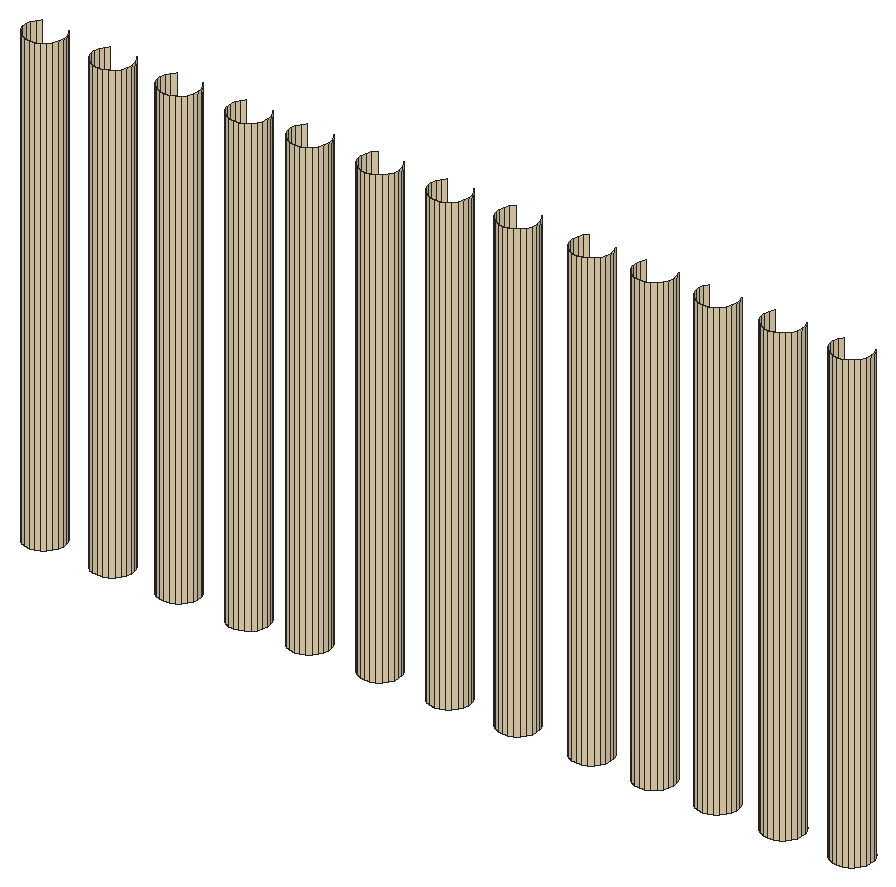
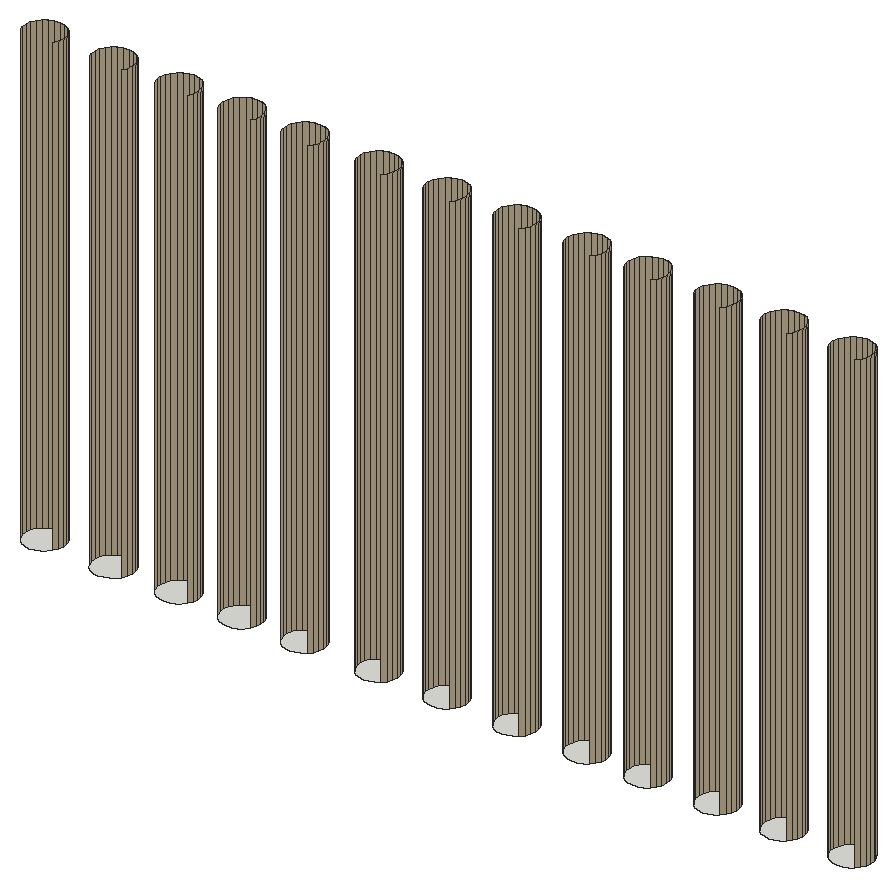
# SketchUp Ruby script. Lengths in inches.
U = 1.inch
M = Sketchup.active_model
def pt(a) = Geom::Point3d.new(a.map { |v| v * U })
def face(e, loops, mat)
  f = e.add_face(loops[0].map { |a| pt(a) })
  loops[1..].each { |l| e.add_face(l.map { |a| pt(a) }).erase! }
  f.material = f.back_material = mat if mat
  f
end
# faces: each face lists its corners as indices into pts; further lists are holes
def faces(e, pts, list, mat = nil) = list.each { |f| face(e, (f[0].is_a?(Array) ? f : [f]).map { |l| l.map { |i| pts[i] } }, mat) }
# xy, xz, yz: faces in a plane at the given z, y or x. An outline is a flat list of corners, or four numbers for a rectangle; further outlines are holes
def ring(l) = l.size == 4 ? [[l[0], l[1]], [l[2], l[1]], [l[2], l[3]], [l[0], l[3]]] : l.each_slice(2).to_a
def flat(e, list, mat, &to3) = list.each { |f| face(e, (f[0].is_a?(Array) ? f : [f]).map { |l| ring(l).map { |u, v| to3.(u, v) } }, mat) }
def xy(e, z, list, mat = nil) = flat(e, list, mat) { |x, y| [x, y, z] }
def xz(e, y, list, mat = nil) = flat(e, list, mat) { |x, z| [x, y, z] }
def yz(e, x, list, mat = nil) = flat(e, list, mat) { |y, z| [x, y, z] }
def lines(e, pts, list) = list.each { |a, b| e.add_line(pt(pts[a]), pt(pts[b])) }
# prism: a flat outline (further loops are holes) pulled along v
def prism(e, loops, v, mat = nil)
  f = face(e, loops, mat); d = Geom::Vector3d.new(v.map { |x| x * U })
  f.pushpull(f.normal.samedirection?(d) ? d.length : -d.length)
end
def box(e, o, s, mat = nil) = prism(e, [[o, [o[0] + s[0], o[1], o[2]], [o[0] + s[0], o[1] + s[1], o[2]], [o[0], o[1] + s[1], o[2]]]], [0, 0, s[2]], mat)
def at(x, y, z, deg = 0) = Geom::Transformation.translation(pt([x, y, z])) * Geom::Transformation.rotation(ORIGIN, Z_AXIS, deg.degrees)
def axes(o, x, y, z) = Geom::Transformation.new([*x, 0, *y, 0, *z, 0, *pt(o).to_a, 1])
def part(name) = M.definitions.add(name)
# library, detail: a bought-in or finely detailed component or shape, given as its bounding box
def library(name, o, s) = part(name).tap { |d| box(d.entities, o, s) }
def detail(e, o, s) = box(e.add_group.entities, o, s)
def put(e, d, t, mat = nil) = e.add_instance(d, t).tap { |i| i.material = mat if mat }
def group(e, t, mat = nil) = e.add_group.tap { |g| g.transformation = t; g.material = mat if mat }.entities
root = M.entities
M.materials.add("[Quartz Light Brown]").color = [242, 223, 185]
xy(root,566.75,[[491.82,18.95,491.37,19.01,490.94,19.18,490.58,19.46,490.3,19.83,490.13,20.25,490.07,20.7,490.13,21.15,490.3,21.58,490.58,21.9375,490.94,22.22,491.37,22.39,491.82,22.45,492.27,22.39,492.69,22.22,493.06,21.9375,493.33,21.58,493.51,21.15,493.57,20.7,493.51,20.25,493.33,19.83,493.06,19.46,492.69,19.18,492.27,19.01],[498.13,18.95,497.68,19.01,497.26,19.18,496.89,19.46,496.62,19.83,496.44,20.25,496.38,20.7,496.44,21.15,496.62,21.58,496.89,21.9375,497.26,22.22,497.68,22.39,498.13,22.45,498.58,22.39,499.01,22.22,499.37,21.9375,499.65,21.58,499.82,21.15,499.88,20.7,499.82,20.25,499.65,19.83,499.37,19.46,499.01,19.18,498.58,19.01],[504.26,18.95,503.8,19.01,503.38,19.18,503.02,19.46,502.74,19.83,502.57,20.25,502.51,20.7,502.57,21.15,502.74,21.58,503.02,21.9375,503.38,22.22,503.8,22.39,504.26,22.45,504.71,22.39,505.13,22.22,505.49,21.9375,505.77,21.58,505.95,21.15,506.01,20.7,505.95,20.25,505.77,19.83,505.49,19.46,505.13,19.18,504.71,19.01],[510.69,18.95,510.24,19.01,509.82,19.18,509.46,19.46,509.18,19.83,509,20.25,508.94,20.7,509,21.15,509.18,21.58,509.46,21.9375,509.82,22.22,510.24,22.39,510.69,22.45,511.15,22.39,511.57,22.22,511.93,21.9375,512.21,21.58,512.38,21.15,512.44,20.7,512.38,20.25,512.21,19.83,511.93,19.46,511.57,19.18,511.15,19.01],[516.32,18.95,515.87,19.01,515.44,19.18,515.08,19.46,514.8,19.83,514.63,20.25,514.57,20.7,514.63,21.15,514.8,21.58,515.08,21.9375,515.44,22.22,515.87,22.39,516.32,22.45,516.77,22.39,517.19,22.22,517.56,21.9375,517.83,21.58,518.01,21.15,518.07,20.7,518.01,20.25,517.83,19.83,517.56,19.46,517.19,19.18,516.77,19.01],
  [522.82,18.95,522.37,19.01,521.94,19.18,521.58,19.46,521.3,19.83,521.13,20.25,521.07,20.7,521.13,21.15,521.3,21.58,521.58,21.9375,521.94,22.22,522.37,22.39,522.82,22.45,523.27,22.39,523.69,22.22,524.06,21.9375,524.33,21.58,524.51,21.15,524.57,20.7,524.51,20.25,524.33,19.83,524.06,19.46,523.69,19.18,523.27,19.01],[529.26,18.95,528.8,19.01,528.38,19.18,528.02,19.46,527.74,19.83,527.57,20.25,527.51,20.7,527.57,21.15,527.74,21.58,528.02,21.9375,528.38,22.22,528.8,22.39,529.26,22.45,529.71,22.39,530.13,22.22,530.49,21.9375,530.77,21.58,530.95,21.15,531.01,20.7,530.95,20.25,530.77,19.83,530.49,19.46,530.13,19.18,529.71,19.01],[535.57,18.95,535.12,19.01,534.69,19.18,534.33,19.46,534.05,19.83,533.88,20.25,533.82,20.7,533.88,21.15,534.05,21.58,534.33,21.9375,534.69,22.22,535.12,22.39,535.57,22.45,536.02,22.39,536.44,22.22,536.81,21.9375,537.08,21.58,537.26,21.15,537.32,20.7,537.26,20.25,537.08,19.83,536.81,19.46,536.44,19.18,536.02,19.01],[542.38,18.95,541.93,19.01,541.51,19.18,541.14,19.46,540.87,19.83,540.69,20.25,540.63,20.7,540.69,21.15,540.87,21.58,541.14,21.9375,541.51,22.22,541.93,22.39,542.38,22.45,542.83,22.39,543.26,22.22,543.62,21.9375,543.9,21.58,544.07,21.15,544.13,20.7,544.07,20.25,543.9,19.83,543.62,19.46,543.26,19.18,542.83,19.01],[548.19,18.95,547.74,19.01,547.32,19.18,546.96,19.46,546.68,19.83,546.5,20.25,546.44,20.7,546.5,21.15,546.68,21.58,546.96,21.9375,547.32,22.22,547.74,22.39,548.19,22.45,548.65,22.39,549.07,22.22,549.43,21.9375,549.71,21.58,549.88,21.15,549.94,20.7,549.88,20.25,549.71,19.83,549.43,19.46,549.07,19.18,548.65,19.01],
  [554.01,18.95,553.55,19.01,553.13,19.18,552.77,19.46,552.49,19.83,552.32,20.25,552.26,20.7,552.32,21.15,552.49,21.58,552.77,21.9375,553.13,22.22,553.55,22.39,554.01,22.45,554.46,22.39,554.88,22.22,555.24,21.9375,555.52,21.58,555.7,21.15,555.76,20.7,555.7,20.25,555.52,19.83,555.24,19.46,554.88,19.18,554.46,19.01],[560.07,18.95,559.62,19.01,559.19,19.18,558.83,19.46,558.55,19.83,558.38,20.25,558.32,20.7,558.38,21.15,558.55,21.58,558.83,21.9375,559.19,22.22,559.62,22.39,560.07,22.45,560.52,22.39,560.94,22.22,561.31,21.9375,561.58,21.58,561.76,21.15,561.82,20.7,561.76,20.25,561.58,19.83,561.31,19.46,560.94,19.18,560.52,19.01],[566.44,18.95,565.99,19.01,565.57,19.18,565.21,19.46,564.93,19.83,564.75,20.25,564.69,20.7,564.75,21.15,564.93,21.58,565.21,21.9375,565.57,22.22,565.99,22.39,566.44,22.45,566.9,22.39,567.32,22.22,567.68,21.9375,567.96,21.58,568.13,21.15,568.19,20.7,568.13,20.25,567.96,19.83,567.68,19.46,567.32,19.18,566.9,19.01]])
p = [[490.94,19.18,566.75],[491.37,19.01,566.75],[491.37,19.01,608.75],[490.94,19.18,608.75],[491.82,18.95,566.75],[491.82,18.95,608.75],
  [492.27,19.01,566.75],[492.27,19.01,608.75],[492.69,19.18,566.75],[492.69,19.18,608.75],[497.26,19.18,566.75],[497.68,19.01,566.75],
  [497.68,19.01,608.75],[497.26,19.18,608.75],[498.13,18.95,566.75],[498.13,18.95,608.75],[498.58,19.01,566.75],[498.58,19.01,608.75],
  [499.01,19.18,566.75],[499.01,19.18,608.75],[503.38,19.18,566.75],[503.8,19.01,566.75],[503.8,19.01,608.75],[503.38,19.18,608.75],
  [504.26,18.95,566.75],[504.26,18.95,608.75],[504.71,19.01,566.75],[504.71,19.01,608.75],[505.13,19.18,566.75],[505.13,19.18,608.75],
  [509.82,19.18,566.75],[510.24,19.01,566.75],[510.24,19.01,608.75],[509.82,19.18,608.75],[510.69,18.95,566.75],[510.69,18.95,608.75],
  [511.15,19.01,566.75],[511.15,19.01,608.75],[511.57,19.18,566.75],[511.57,19.18,608.75],[515.44,19.18,566.75],[515.87,19.01,566.75],
  [515.87,19.01,608.75],[515.44,19.18,608.75],[516.32,18.95,566.75],[516.32,18.95,608.75],[516.77,19.01,566.75],[516.77,19.01,608.75],
  [517.19,19.18,566.75],[517.19,19.18,608.75],[521.94,19.18,566.75],[522.37,19.01,566.75],[522.37,19.01,608.75],[521.94,19.18,608.75],
  [522.82,18.95,566.75],[522.82,18.95,608.75],[523.27,19.01,566.75],[523.27,19.01,608.75],[523.69,19.18,566.75],[523.69,19.18,608.75],
  [528.38,19.18,566.75],[528.8,19.01,566.75],[528.8,19.01,608.75],[528.38,19.18,608.75],[529.26,18.95,566.75],[529.26,18.95,608.75],
  [529.71,19.01,566.75],[529.71,19.01,608.75],[530.13,19.18,566.75],[530.13,19.18,608.75],[534.69,19.18,566.75],[535.12,19.01,566.75],
  [535.12,19.01,608.75],[534.69,19.18,608.75],[535.57,18.95,566.75],[535.57,18.95,608.75],[536.02,19.01,566.75],[536.02,19.01,608.75],
  [536.44,19.18,566.75],[536.44,19.18,608.75],[541.51,19.18,566.75],[541.93,19.01,566.75],[541.93,19.01,608.75],[541.51,19.18,608.75],
  [542.38,18.95,566.75],[542.38,18.95,608.75],[542.83,19.01,566.75],[542.83,19.01,608.75],[543.26,19.18,566.75],[543.26,19.18,608.75],
  [547.32,19.18,566.75],[547.74,19.01,566.75],[547.74,19.01,608.75],[547.32,19.18,608.75],[548.19,18.95,566.75],[548.19,18.95,608.75],
  [548.65,19.01,566.75],[548.65,19.01,608.75],[549.07,19.18,566.75],[549.07,19.18,608.75],[553.13,19.18,566.75],[553.55,19.01,566.75],
  [553.55,19.01,608.75],[553.13,19.18,608.75],[554.01,18.95,566.75],[554.01,18.95,608.75],[554.46,19.01,566.75],[554.46,19.01,608.75],
  [554.88,19.18,566.75],[554.88,19.18,608.75],[559.19,19.18,566.75],[559.62,19.01,566.75],[559.62,19.01,608.75],[559.19,19.18,608.75],
  [560.07,18.95,566.75],[560.07,18.95,608.75],[560.52,19.01,566.75],[560.52,19.01,608.75],[560.94,19.18,566.75],[560.94,19.18,608.75],
  [565.57,19.18,566.75],[565.99,19.01,566.75],[565.99,19.01,608.75],[565.57,19.18,608.75],[566.44,18.95,566.75],[566.44,18.95,608.75],
  [566.9,19.01,566.75],[566.9,19.01,608.75],[567.32,19.18,566.75],[567.32,19.18,608.75],[490.58,19.46,566.75],[490.58,19.46,608.75],
  [493.06,19.46,566.75],[493.06,19.46,608.75],[496.89,19.46,566.75],[496.89,19.46,608.75],[499.37,19.46,566.75],[499.37,19.46,608.75],
  [503.02,19.46,566.75],[503.02,19.46,608.75],[505.49,19.46,566.75],[505.49,19.46,608.75],[509.46,19.46,566.75],[509.46,19.46,608.75],
  [511.93,19.46,566.75],[511.93,19.46,608.75],[515.08,19.46,566.75],[515.08,19.46,608.75],[517.56,19.46,566.75],[517.56,19.46,608.75],
  [521.58,19.46,566.75],[521.58,19.46,608.75],[524.06,19.46,566.75],[524.06,19.46,608.75],[528.02,19.46,566.75],[528.02,19.46,608.75],
  [530.49,19.46,566.75],[530.49,19.46,608.75],[534.33,19.46,566.75],[534.33,19.46,608.75],[536.81,19.46,566.75],[536.81,19.46,608.75],
  [541.14,19.46,566.75],[541.14,19.46,608.75],[543.62,19.46,566.75],[543.62,19.46,608.75],[546.96,19.46,566.75],[546.96,19.46,608.75],
  [549.43,19.46,566.75],[549.43,19.46,608.75],[552.77,19.46,566.75],[552.77,19.46,608.75],[555.24,19.46,566.75],[555.24,19.46,608.75],
  [558.83,19.46,566.75],[558.83,19.46,608.75],[561.31,19.46,566.75],[561.31,19.46,608.75],[565.21,19.46,566.75],[565.21,19.46,608.75],
  [567.68,19.46,566.75],[567.68,19.46,608.75],[490.3,19.83,566.75],[490.3,19.83,608.75],[493.33,19.83,566.75],[493.33,19.83,608.75],
  [496.62,19.83,566.75],[496.62,19.83,608.75],[499.65,19.83,566.75],[499.65,19.83,608.75],[502.74,19.83,566.75],[502.74,19.83,608.75],
  [505.77,19.83,566.75],[505.77,19.83,608.75],[509.18,19.83,566.75],[509.18,19.83,608.75],[512.21,19.83,566.75],[512.21,19.83,608.75],
  [514.8,19.83,566.75],[514.8,19.83,608.75],[517.83,19.83,566.75],[517.83,19.83,608.75],[521.3,19.83,566.75],[521.3,19.83,608.75],
  [524.33,19.83,566.75],[524.33,19.83,608.75],[527.74,19.83,566.75],[527.74,19.83,608.75],[530.77,19.83,566.75],[530.77,19.83,608.75],
  [534.05,19.83,566.75],[534.05,19.83,608.75],[537.08,19.83,566.75],[537.08,19.83,608.75],[540.87,19.83,566.75],[540.87,19.83,608.75],
  [543.9,19.83,566.75],[543.9,19.83,608.75],[546.68,19.83,566.75],[546.68,19.83,608.75],[549.71,19.83,566.75],[549.71,19.83,608.75],
  [552.49,19.83,566.75],[552.49,19.83,608.75],[555.52,19.83,566.75],[555.52,19.83,608.75],[558.55,19.83,566.75],[558.55,19.83,608.75],
  [561.58,19.83,566.75],[561.58,19.83,608.75],[564.93,19.83,566.75],[564.93,19.83,608.75],[567.96,19.83,566.75],[567.96,19.83,608.75],
  [490.13,20.25,566.75],[490.13,20.25,608.75],[493.51,20.25,566.75],[493.51,20.25,608.75],[496.44,20.25,566.75],[496.44,20.25,608.75],
  [499.82,20.25,566.75],[499.82,20.25,608.75],[502.57,20.25,566.75],[502.57,20.25,608.75],[505.95,20.25,566.75],[505.95,20.25,608.75],
  [509,20.25,566.75],[509,20.25,608.75],[512.38,20.25,566.75],[512.38,20.25,608.75],[514.63,20.25,566.75],[514.63,20.25,608.75],
  [518.01,20.25,566.75],[518.01,20.25,608.75],[521.13,20.25,566.75],[521.13,20.25,608.75],[524.51,20.25,566.75],[524.51,20.25,608.75],
  [527.57,20.25,566.75],[527.57,20.25,608.75],[530.95,20.25,566.75],[530.95,20.25,608.75],[533.88,20.25,566.75],[533.88,20.25,608.75],
  [537.26,20.25,566.75],[537.26,20.25,608.75],[540.69,20.25,566.75],[540.69,20.25,608.75],[544.07,20.25,566.75],[544.07,20.25,608.75],
  [546.5,20.25,566.75],[546.5,20.25,608.75],[549.88,20.25,566.75],[549.88,20.25,608.75],[552.32,20.25,566.75],[552.32,20.25,608.75],
  [555.7,20.25,566.75],[555.7,20.25,608.75],[558.38,20.25,566.75],[558.38,20.25,608.75],[561.76,20.25,566.75],[561.76,20.25,608.75],
  [564.75,20.25,566.75],[564.75,20.25,608.75],[568.13,20.25,566.75],[568.13,20.25,608.75],[490.07,20.7,566.75],[490.07,20.7,608.75],
  [493.57,20.7,566.75],[493.57,20.7,608.75],[496.38,20.7,566.75],[496.38,20.7,608.75],[499.88,20.7,566.75],[499.88,20.7,608.75],
  [502.51,20.7,566.75],[502.51,20.7,608.75],[506.01,20.7,566.75],[506.01,20.7,608.75],[508.94,20.7,566.75],[508.94,20.7,608.75],
  [512.44,20.7,566.75],[512.44,20.7,608.75],[514.57,20.7,566.75],[514.57,20.7,608.75],[518.07,20.7,566.75],[518.07,20.7,608.75],
  [521.07,20.7,566.75],[521.07,20.7,608.75],[524.57,20.7,566.75],[524.57,20.7,608.75],[527.51,20.7,566.75],[527.51,20.7,608.75],
  [531.01,20.7,566.75],[531.01,20.7,608.75],[533.82,20.7,566.75],[533.82,20.7,608.75],[537.32,20.7,566.75],[537.32,20.7,608.75],
  [540.63,20.7,566.75],[540.63,20.7,608.75],[544.13,20.7,566.75],[544.13,20.7,608.75],[546.44,20.7,566.75],[546.44,20.7,608.75],
  [549.94,20.7,566.75],[549.94,20.7,608.75],[552.26,20.7,566.75],[552.26,20.7,608.75],[555.76,20.7,566.75],[555.76,20.7,608.75],
  [558.32,20.7,566.75],[558.32,20.7,608.75],[561.82,20.7,566.75],[561.82,20.7,608.75],[564.69,20.7,566.75],[564.69,20.7,608.75],
  [568.19,20.7,566.75],[568.19,20.7,608.75],[490.13,21.15,566.75],[490.13,21.15,608.75],[493.51,21.15,566.75],[493.51,21.15,608.75],
  [496.44,21.15,566.75],[496.44,21.15,608.75],[499.82,21.15,566.75],[499.82,21.15,608.75],[502.57,21.15,566.75],[502.57,21.15,608.75],
  [505.95,21.15,566.75],[505.95,21.15,608.75],[509,21.15,566.75],[509,21.15,608.75],[512.38,21.15,566.75],[512.38,21.15,608.75],
  [514.63,21.15,566.75],[514.63,21.15,608.75],[518.01,21.15,566.75],[518.01,21.15,608.75],[521.13,21.15,566.75],[521.13,21.15,608.75],
  [524.51,21.15,566.75],[524.51,21.15,608.75],[527.57,21.15,566.75],[527.57,21.15,608.75],[530.95,21.15,566.75],[530.95,21.15,608.75],
  [533.88,21.15,566.75],[533.88,21.15,608.75],[537.26,21.15,566.75],[537.26,21.15,608.75],[540.69,21.15,566.75],[540.69,21.15,608.75],
  [544.07,21.15,566.75],[544.07,21.15,608.75],[546.5,21.15,566.75],[546.5,21.15,608.75],[549.88,21.15,566.75],[549.88,21.15,608.75],
  [552.32,21.15,566.75],[552.32,21.15,608.75],[555.7,21.15,566.75],[555.7,21.15,608.75],[558.38,21.15,566.75],[558.38,21.15,608.75],
  [561.76,21.15,566.75],[561.76,21.15,608.75],[564.75,21.15,566.75],[564.75,21.15,608.75],[568.13,21.15,566.75],[568.13,21.15,608.75],
  [490.3,21.58,566.75],[490.3,21.58,608.75],[493.33,21.58,566.75],[493.33,21.58,608.75],[496.62,21.58,566.75],[496.62,21.58,608.75],
  [499.65,21.58,566.75],[499.65,21.58,608.75],[502.74,21.58,566.75],[502.74,21.58,608.75],[505.77,21.58,566.75],[505.77,21.58,608.75],
  [509.18,21.58,566.75],[509.18,21.58,608.75],[512.21,21.58,566.75],[512.21,21.58,608.75],[514.8,21.58,566.75],[514.8,21.58,608.75],
  [517.83,21.58,566.75],[517.83,21.58,608.75],[521.3,21.58,566.75],[521.3,21.58,608.75],[524.33,21.58,566.75],[524.33,21.58,608.75],
  [527.74,21.58,566.75],[527.74,21.58,608.75],[530.77,21.58,566.75],[530.77,21.58,608.75],[534.05,21.58,566.75],[534.05,21.58,608.75],
  [537.08,21.58,566.75],[537.08,21.58,608.75],[540.87,21.58,566.75],[540.87,21.58,608.75],[543.9,21.58,566.75],[543.9,21.58,608.75],
  [546.68,21.58,566.75],[546.68,21.58,608.75],[549.71,21.58,566.75],[549.71,21.58,608.75],[552.49,21.58,566.75],[552.49,21.58,608.75],
  [555.52,21.58,566.75],[555.52,21.58,608.75],[558.55,21.58,566.75],[558.55,21.58,608.75],[561.58,21.58,566.75],[561.58,21.58,608.75],
  [564.93,21.58,566.75],[564.93,21.58,608.75],[567.96,21.58,566.75],[567.96,21.58,608.75],[490.58,21.9375,566.75],[490.58,21.9375,608.75],
  [493.06,21.9375,566.75],[493.06,21.9375,608.75],[496.89,21.9375,566.75],[496.89,21.9375,608.75],[499.37,21.9375,566.75],[499.37,21.9375,608.75],
  [503.02,21.9375,566.75],[503.02,21.9375,608.75],[505.49,21.9375,566.75],[505.49,21.9375,608.75],[509.46,21.9375,566.75],[509.46,21.9375,608.75],
  [511.93,21.9375,566.75],[511.93,21.9375,608.75],[515.08,21.9375,566.75],[515.08,21.9375,608.75],[517.56,21.9375,566.75],[517.56,21.9375,608.75],
  [521.58,21.9375,566.75],[521.58,21.9375,608.75],[524.06,21.9375,566.75],[524.06,21.9375,608.75],[528.02,21.9375,566.75],[528.02,21.9375,608.75],
  [530.49,21.9375,566.75],[530.49,21.9375,608.75],[534.33,21.9375,566.75],[534.33,21.9375,608.75],[536.81,21.9375,566.75],[536.81,21.9375,608.75],
  [541.14,21.9375,566.75],[541.14,21.9375,608.75]]
faces(root,p,[[0,1,2,3],[1,4,5,2],[4,6,7,5],[6,8,9,7],[10,11,12,13],[11,14,15,12],[14,16,17,15],[16,18,19,17],
  [20,21,22,23],[21,24,25,22],[24,26,27,25],[26,28,29,27],[30,31,32,33],[31,34,35,32],[34,36,37,35],[36,38,39,37],
  [40,41,42,43],[41,44,45,42],[44,46,47,45],[46,48,49,47],[50,51,52,53],[51,54,55,52],[54,56,57,55],[56,58,59,57],
  [60,61,62,63],[61,64,65,62],[64,66,67,65],[66,68,69,67],[70,71,72,73],[71,74,75,72],[74,76,77,75],[76,78,79,77],
  [80,81,82,83],[81,84,85,82],[84,86,87,85],[86,88,89,87],[90,91,92,93],[91,94,95,92],[94,96,97,95],[96,98,99,97],
  [100,101,102,103],[101,104,105,102],[104,106,107,105],[106,108,109,107],[110,111,112,113],[111,114,115,112],[114,116,117,115],[116,118,119,117],
  [120,121,122,123],[121,124,125,122],[124,126,127,125],[126,128,129,127],[130,0,3,131],[8,132,133,9],[134,10,13,135],[18,136,137,19],
  [138,20,23,139],[28,140,141,29],[142,30,33,143],[38,144,145,39],[146,40,43,147],[48,148,149,49],[150,50,53,151],[58,152,153,59],
  [154,60,63,155],[68,156,157,69],[158,70,73,159],[78,160,161,79],[162,80,83,163],[88,164,165,89],[166,90,93,167],[98,168,169,99],
  [170,100,103,171],[108,172,173,109],[174,110,113,175],[118,176,177,119],[178,120,123,179],[128,180,181,129],[182,130,131,183],[132,184,185,133],
  [186,134,135,187],[136,188,189,137],[190,138,139,191],[140,192,193,141],[194,142,143,195],[144,196,197,145],[198,146,147,199],[148,200,201,149],
  [202,150,151,203],[152,204,205,153],[206,154,155,207],[156,208,209,157],[210,158,159,211],[160,212,213,161],[214,162,163,215],[164,216,217,165],
  [218,166,167,219],[168,220,221,169],[222,170,171,223],[172,224,225,173],[226,174,175,227],[176,228,229,177],[230,178,179,231],[180,232,233,181],
  [234,182,183,235],[184,236,237,185],[238,186,187,239],[188,240,241,189],[242,190,191,243],[192,244,245,193],[246,194,195,247],[196,248,249,197],
  [250,198,199,251],[200,252,253,201],[254,202,203,255],[204,256,257,205],[258,206,207,259],[208,260,261,209],[262,210,211,263],[212,264,265,213],
  [266,214,215,267],[216,268,269,217],[270,218,219,271],[220,272,273,221],[274,222,223,275],[224,276,277,225],[278,226,227,279],[228,280,281,229],
  [282,230,231,283],[232,284,285,233],[286,234,235,287],[236,288,289,237],[290,238,239,291],[240,292,293,241],[294,242,243,295],[244,296,297,245],
  [298,246,247,299],[248,300,301,249],[302,250,251,303],[252,304,305,253],[306,254,255,307],[256,308,309,257],[310,258,259,311],[260,312,313,261],
  [314,262,263,315],[264,316,317,265],[318,266,267,319],[268,320,321,269],[322,270,271,323],[272,324,325,273],[326,274,275,327],[276,328,329,277],
  [330,278,279,331],[280,332,333,281],[334,282,283,335],[284,336,337,285],[338,286,287,339],[288,340,341,289],[342,290,291,343],[292,344,345,293],
  [346,294,295,347],[296,348,349,297],[350,298,299,351],[300,352,353,301],[354,302,303,355],[304,356,357,305],[358,306,307,359],[308,360,361,309],
  [362,310,311,363],[312,364,365,313],[366,314,315,367],[316,368,369,317],[370,318,319,371],[320,372,373,321],[374,322,323,375],[324,376,377,325],
  [378,326,327,379],[328,380,381,329],[382,330,331,383],[332,384,385,333],[386,334,335,387],[336,388,389,337],[390,338,339,391],[340,392,393,341],
  [394,342,343,395],[344,396,397,345],[398,346,347,399],[348,400,401,349],[402,350,351,403],[352,404,405,353],[406,354,355,407],[356,408,409,357],
  [410,358,359,411],[360,412,413,361],[414,362,363,415],[364,416,417,365],[418,366,367,419],[368,420,421,369],[422,370,371,423],[372,424,425,373],
  [426,374,375,427],[376,428,429,377],[430,378,379,431],[380,432,433,381],[434,382,383,435],[384,436,437,385],[438,386,387,439],[388,440,441,389],
  [442,390,391,443],[392,444,445,393],[446,394,395,447],[396,448,449,397],[450,398,399,451],[400,452,453,401],[454,402,403,455],[404,456,457,405],
  [458,406,407,459],[408,460,461,409],[462,410,411,463],[412,464,465,413],[466,414,415,467],[416,468,469,417],[470,418,419,471],[420,472,473,421],
  [474,422,423,475]],"[Quartz Light Brown]")
